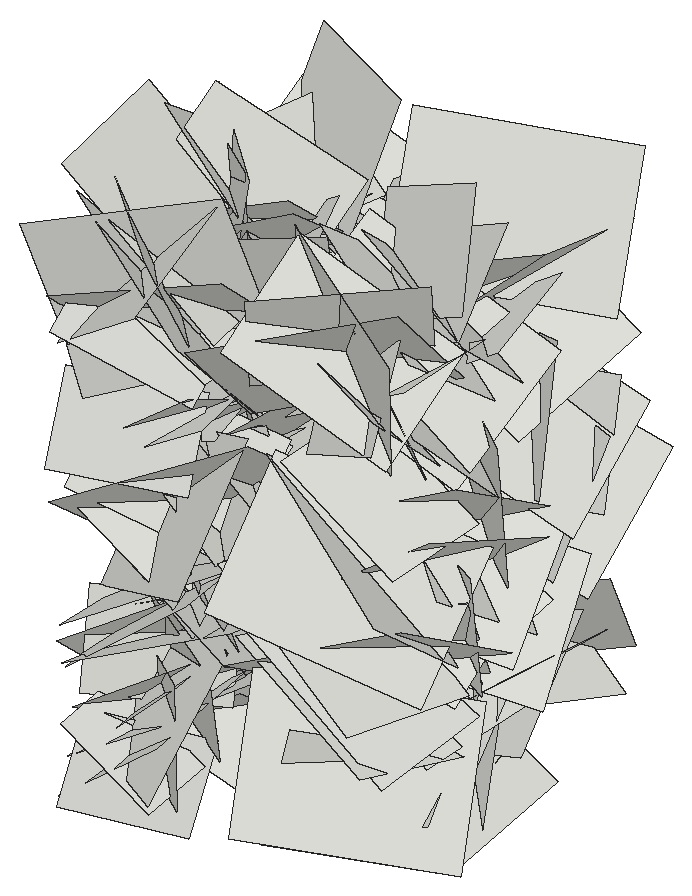
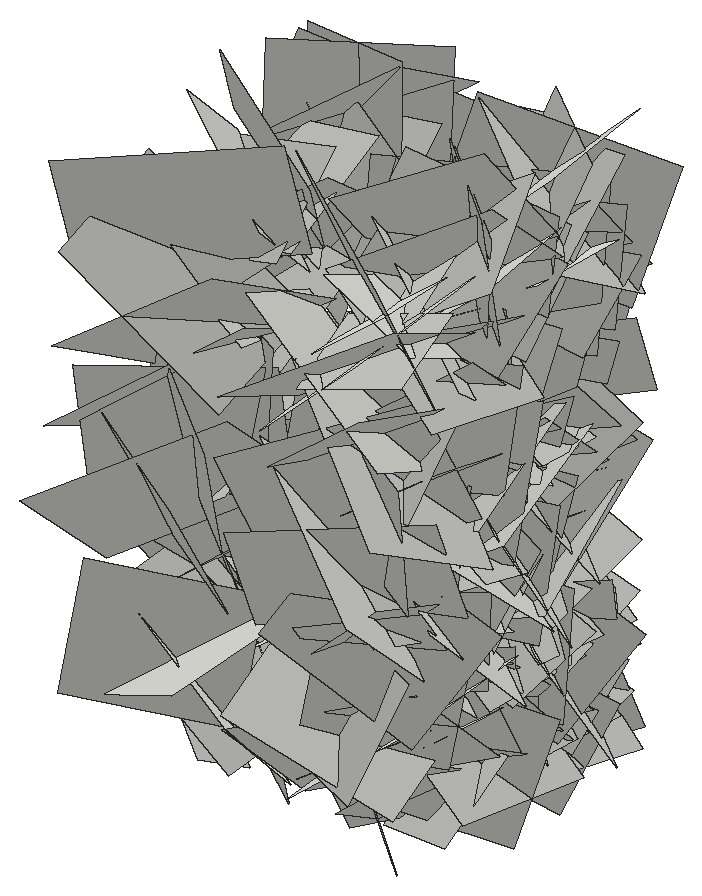
# SketchUp Ruby script. Lengths in inches.
U = 1.inch
M = Sketchup.active_model
def pt(a) = Geom::Point3d.new(a.map { |v| v * U })
def face(e, loops, mat)
  f = e.add_face(loops[0].map { |a| pt(a) })
  loops[1..].each { |l| e.add_face(l.map { |a| pt(a) }).erase! }
  f.material = f.back_material = mat if mat
  f
end
# faces: each face lists its corners as indices into pts; further lists are holes
def faces(e, pts, list, mat = nil) = list.each { |f| face(e, (f[0].is_a?(Array) ? f : [f]).map { |l| l.map { |i| pts[i] } }, mat) }
# xy, xz, yz: faces in a plane at the given z, y or x. An outline is a flat list of corners, or four numbers for a rectangle; further outlines are holes
def ring(l) = l.size == 4 ? [[l[0], l[1]], [l[2], l[1]], [l[2], l[3]], [l[0], l[3]]] : l.each_slice(2).to_a
def flat(e, list, mat, &to3) = list.each { |f| face(e, (f[0].is_a?(Array) ? f : [f]).map { |l| ring(l).map { |u, v| to3.(u, v) } }, mat) }
def xy(e, z, list, mat = nil) = flat(e, list, mat) { |x, y| [x, y, z] }
def xz(e, y, list, mat = nil) = flat(e, list, mat) { |x, z| [x, y, z] }
def yz(e, x, list, mat = nil) = flat(e, list, mat) { |y, z| [x, y, z] }
def lines(e, pts, list) = list.each { |a, b| e.add_line(pt(pts[a]), pt(pts[b])) }
# prism: a flat outline (further loops are holes) pulled along v
def prism(e, loops, v, mat = nil)
  f = face(e, loops, mat); d = Geom::Vector3d.new(v.map { |x| x * U })
  f.pushpull(f.normal.samedirection?(d) ? d.length : -d.length)
end
def box(e, o, s, mat = nil) = prism(e, [[o, [o[0] + s[0], o[1], o[2]], [o[0] + s[0], o[1] + s[1], o[2]], [o[0], o[1] + s[1], o[2]]]], [0, 0, s[2]], mat)
def at(x, y, z, deg = 0) = Geom::Transformation.translation(pt([x, y, z])) * Geom::Transformation.rotation(ORIGIN, Z_AXIS, deg.degrees)
def axes(o, x, y, z) = Geom::Transformation.new([*x, 0, *y, 0, *z, 0, *pt(o).to_a, 1])
def part(name) = M.definitions.add(name)
# library, detail: a bought-in or finely detailed component or shape, given as its bounding box
def library(name, o, s) = part(name).tap { |d| box(d.entities, o, s) }
def detail(e, o, s) = box(e.add_group.entities, o, s)
def put(e, d, t, mat = nil) = e.add_instance(d, t).tap { |i| i.material = mat if mat }
def group(e, t, mat = nil) = e.add_group.tap { |g| g.transformation = t; g.material = mat if mat }.entities
root = M.entities
c1 = part("Component\#6")
p = [[0.01,0,0],[0,3.24,4.54],[4.32,3.24,4.54],[4.33,0,0]]
faces(c1.entities,p,[[0,1,2,3]])
put(root,c1,axes([410.71,188.38,23.95],[-0.14683,-0.05211,-1.06804],[-0.1506,-1.06652,0.07046],[1.12342,-0.14978,-0.13015]))
put(root,c1,axes([414.68,187.95,18.35],[0.24952,-0.85217,0.60628],[0.01294,0.62364,0.87183],[-1.1085,-0.18454,0.14665]))
put(root,c1,axes([414.68,184.68,7.1],[0.07537,-0.21143,-0.85755],[0.01444,-0.85996,0.21315],[-0.93612,-0.03029,-0.06575]))
put(root,c1,axes([410.71,184.16,21.8125],[-0.07155,0.99261,-0.10082],[-0.11355,-0.10768,-0.9884],[1.05147,0.05592,-0.1136]))
put(root,c1,axes([410.71,192.04,5.47],[-0.24252,-0.79203,0.72828],[-0.0092,0.7459,0.80846],[1.14049,-0.1624,0.16139]))
put(root,c1,axes([410.71,189.65,5.54],[0.06955,0.77959,0.08211],[0.00823,0.08175,-0.78235],[0.8309,-0.06607,0.00087]))
put(root,c1,axes([410.71,189.86,21.06],[-0.09411,0.75469,-0.30292],[0.23058,-0.27158,-0.74036],[0.83059,0.16091,0.17121]))
put(root,c1,axes([410.71,184.33,2.33],[-0.23495,-0.78095,0.69461],[0.033,0.70481,0.80235],[1.10738,-0.18669,0.12346]))
put(root,c1,axes([414.68,182.875,15.8],[0.04284,-0.30855,-0.78276],[0.017,-0.78324,0.30957],[-0.8917,-0.02976,-0.0317]))
put(root,c1,axes([414.68,183.91,5.17],[0.1157,0.58195,-0.7538],[0.08085,-0.76164,-0.57696],[-1.0062,0.00571,-0.13304]))
put(root,c1,axes([414.68,180.19,4.07],[-0.08532,0.68038,-0.07405],[-0.04058,-0.07892,-0.68351],[-0.72433,-0.07573,0.04702]))
put(root,c1,axes([414.68,182.98,9.92],[-0.09782,-0.62966,-0.10425],[-0.08997,-0.09229,0.63256],[-0.67052,0.10424,-0.06967]))
put(root,c1,axes([414.68,190.84,12.42],[-0.00848,-0.77925,-0.15089],[0.03038,-0.15108,0.77873],[-0.8408,0.0024,0.02966]))
put(root,c1,axes([414.68,191.35,2.27],[0.06694,-0.86655,-0.10749],[0.04783,-0.10439,0.86806],[-0.92435,-0.06816,0.03713]))
put(root,c1,axes([414.68,191.46,9.82],[0.08538,-0.06629,-0.92063],[0.09555,-0.91915,0.07407],[-0.97372,-0.09601,-0.07345]))
put(root,c1,axes([414.68,193.37,9.31],[0.05697,-0.46717,-0.61186],[-0.09106,-0.61316,0.46062],[-0.81091,0.03603,-0.09471]))
put(root,c1,axes([414.68,183.28,17.73],[0.09647,-0.26045,0.74001],[-0.11879,0.73302,0.27177],[-0.82305,-0.13632,0.04751]))
put(root,c1,axes([414.68,185.14,8.49],[-0.08576,-0.66072,-0.04627],[-0.0456,-0.04128,0.66459],[-0.70059,0.08356,-0.03759]))
put(root,c1,axes([414.68,192.03,8.33],[0.03388,0.22508,-0.86549],[0.13142,-0.8588,-0.21876],[-0.93879,-0.1121,-0.06186]))
put(root,c1,axes([410.71,192.08,20.31],[0.05296,-0.67773,-0.30339],[0.1724,-0.2867,0.66724],[0.76797,0.11109,-0.12886]))
put(root,c1,axes([410.71,184.53,11.29],[-0.10396,-0.95246,0.37472],[-0.04499,0.37989,0.95451],[1.084,-0.07558,0.07555]))
put(root,c1,axes([414.68,183.19,13.8],[0.02762,0.65605,0.3231],[-0.06014,0.32414,-0.6536],[-0.77284,-0.00178,0.06241]))
put(root,c1,axes([414.68,185.94,13.1875],[0.12339,0.16979,-0.82402],[-0.01755,-0.83125,-0.17361],[-0.89164,0.03986,-0.11061]))
put(root,c1,axes([414.68,185.26,12.26],[0.159,0.84642,0.10737],[-0.04855,0.11685,-0.85715],[-0.9031,0.14274,0.06498]))
put(root,c1,axes([410.71,181.6,11.88],[0.05183,0.72565,0.67247],[-0.15864,0.67097,-0.71314],[1.03662,0.0664,-0.14276]))
put(root,c1,axes([414.68,192.38,19.24],[-0.04943,-0.7355,0.057],[0.07325,0.05251,0.73407],[-0.77853,0.05163,0.06545]))
put(root,c1,axes([410.71,185.13,2.21],[0.09174,0.69928,0.36],[0.10121,0.35015,-0.7031],[0.82753,-0.12035,0.04608]))
put(root,c1,axes([410.71,185.25,15.47],[0.04372,0.77316,0.71524],[-0.20224,0.70943,-0.75587],[1.09798,0.09988,-0.16771]))
put(root,c1,axes([410.71,183.61,1.59],[0.06331,-0.78644,0.46242],[-0.03597,0.46118,0.7887],[0.96639,0.06869,-0.00094]))
put(root,c1,axes([410.71,186.63,-0.64],[-0.14781,-0.37723,1.01914],[-0.01271,1.02797,0.37886],[1.15185,-0.03706,0.13496]))
put(root,c1,axes([410.71,183.46,7.83],[-0.1867,0.36795,-0.96583],[0.13041,-0.96532,-0.39019],[1.08777,0.17888,-0.11899]))
put(root,c1,axes([414.68,192.83,7.86],[-0.1126,-0.65912,-0.17655],[0.1088,-0.19208,0.65534],[-0.71507,0.07456,0.12751]))
put(root,c1,axes([414.68,183.375,2.21],[-0.01982,-0.33114,-0.74136],[0.16849,-0.7287,0.32148],[-0.84401,-0.13769,0.08159]))
put(root,c1,axes([410.71,187.85,22.99],[0.09057,-0.06637,-0.91857],[-0.07612,-0.92019,0.05981],[0.97325,-0.06579,0.09016]))
put(root,c1,axes([410.71,187.17,12.95],[-0.05814,-0.16279,1.09674],[-0.14666,1.09051,0.15494],[1.1661,0.12904,0.07417]))
put(root,c1,axes([410.71,185.08,2.16],[0.06404,-1.02262,-0.11109],[-0.17979,-0.11966,1.00929],[1.07543,0.04089,0.17535]))
put(root,c1,axes([410.71,180.14,11.99],[-0.0212,0.75168,0.8023],[-0.17372,0.79143,-0.74558],[1.15236,0.13314,-0.09764]))
put(root,c1,axes([414.68,186.92,8.78],[0.10246,-0.30095,0.75916],[0.04625,0.76527,0.29782],[-0.86439,0.00528,0.10592]))
put(root,c1,axes([410.71,191,16.96],[-0.17643,-1.14926,-0.11809],[-0.05518,-0.11173,1.16072],[1.22339,-0.17078,0.03532]))
put(root,c1,axes([410.71,189.57,16.9],[0.06471,0.53395,-0.71324],[0.01751,-0.71546,-0.53421],[0.94426,-0.02333,0.05878]))
put(root,c1,axes([414.68,184.43,15.42],[0.12844,-0.04329,0.74472],[-0.08874,0.74892,0.05716],[-0.78574,-0.09166,0.11528]))
put(root,c1,axes([410.71,179.97,24.47],[-0.23304,1.36821,0.06434],[-0.25904,0.02493,-1.36533],[1.42861,0.2277,-0.23708]))
put(root,c1,axes([414.68,182.67,1.51],[0.02969,-0.72745,-0.10184],[0.03667,-0.1005,0.72735],[-0.77775,-0.03251,0.03041]))
put(root,c1,axes([410.71,190.33,17.67],[0.17424,0.82504,0.17436],[-0.04616,0.18571,-0.83769],[0.89267,-0.15144,-0.07735]))
put(root,c1,axes([410.71,186.72,4.72],[-0.08241,-0.91883,0.29273],[0.13826,0.28096,0.91654],[1.0128,-0.11312,-0.1013]))
put(root,c1,axes([410.71,185.64,19.96],[-0.2349,1.07139,0.39402],[0.08081,0.41437,-1.08385],[1.20734,0.18072,0.1492]))
put(root,c1,axes([414.68,184.54,3.47],[0.05739,0.5962,-0.42459],[0.0201,-0.42675,-0.59681],[-0.77559,0.03305,-0.04688]))
put(root,c1,axes([414.68,189.45,1.42],[-0.1039,0.30381,0.53974],[0.07033,0.54846,-0.29667],[-0.65275,0.01074,-0.11787]))
put(root,c1,axes([410.71,186.9375,3.03],[0.11563,0.62873,-0.58509],[0.05581,-0.59358,-0.62803],[0.90867,-0.04354,0.11303]))
put(root,c1,axes([410.71,184.51,1.15],[-0.01173,-1.06899,-0.22188],[-0.10644,-0.21996,1.06472],[1.15237,-0.0312,0.09608]))
put(root,c1,axes([414.68,183.83,7.3125],[0.02805,0.62389,-0.09529],[-0.05665,-0.09282,-0.62253],[-0.66659,0.03414,0.0489]))
put(root,c1,axes([414.68,183.1,18.89],[0.1435,0.17311,-0.85276],[0.14536,-0.85648,-0.1521],[-0.91084,-0.10941,-0.15862]))
put(root,c1,axes([410.71,187.61,11.62],[-0.28203,-0.58282,-1.12773],[0.01249,-1.15332,0.59327],[1.34554,-0.11146,-0.24188]))
put(root,c1,axes([410.71,184.19,13.53],[0.08078,-0.49886,0.79857],[0.01528,0.8017,0.49945],[0.99796,0.02811,-0.07229]))
put(root,c1,axes([410.71,181.29,16.68],[0.08133,-0.245,0.96212],[-0.05676,0.96256,0.24939],[1.05086,0.07095,-0.06099]))
put(root,c1,axes([414.68,186.0625,6.1],[0.08854,0.52684,0.45627],[-0.00383,0.45985,-0.53032],[-0.73876,0.06076,0.05744]))
put(root,c1,axes([414.68,187.98,11.49],[0.12716,0.81746,0.20835],[0.15,0.18797,-0.81896],[-0.88154,0.1499,-0.10929]))
put(root,c1,axes([410.71,194.3,13.93],[-0.22437,-1.23478,-0.60854],[-0.19245,-0.58527,1.25072],[1.44644,-0.26941,0.07201]))
put(root,c1,axes([410.71,184.41,20.14],[-0.03821,-1.03167,-0.60174],[-0.15497,-0.59368,1.0266],[1.25647,-0.1046,0.10832]))
put(root,c1,axes([414.68,186.3,8.38],[-0.07617,0.47932,0.41871],[0.13681,0.42359,-0.46276],[-0.66062,0.03245,-0.14411]))
put(root,c1,axes([410.71,184.31,4.6],[0.1576,-0.1516,-1.0147],[-0.15202,-1.0183,0.13112],[1.07684,-0.12157,0.16702]))
put(root,c1,axes([410.71,179.32,18.3],[0.15069,0.54422,0.74866],[-0.00735,0.75804,-0.54972],[0.98107,-0.07791,-0.11911]))
put(root,c1,axes([414.68,188.8,6.44],[0.14743,-0.18272,-0.74199],[0.06403,-0.74919,0.19581],[-0.80747,-0.09277,-0.11994]))
put(root,c1,axes([410.71,185.52,6.2],[-0.2751,-0.65276,-1.16933],[-0.03559,-1.18754,0.67037],[1.41909,-0.15632,-0.20987]))
put(root,c1,axes([410.71,181.08,20.02],[-0.00536,1.00575,0.03656],[0.10796,0.03689,-1.00058],[1.06133,0.00133,0.10197]))
put(root,c1,axes([410.71,184.05,20.67],[0.10102,0.73684,0.6989],[-0.04073,0.70408,-0.73707],[1.07574,-0.04254,-0.09354]))
put(root,c1,axes([410.71,191.125,9.45],[-0.23474,-0.88576,-0.93612],[0.00151,-0.95001,0.89856],[1.36608,-0.15116,-0.16185]))
put(root,c1,axes([410.71,185.11,13.22],[0.08906,-0.95701,-0.12674],[0.0585,-0.12225,0.95969],[1.02162,0.09043,-0.0439]))
put(root,c1,axes([410.71,180.4,17.125],[-0.23878,-0.31981,1.17522],[0.15258,1.17979,0.34864],[1.28199,-0.19998,0.17739]))
put(root,c1,axes([410.71,187.48,17.59],[-0.04794,-0.78864,0.66349],[0.19289,0.64758,0.78214],[1.07529,-0.15133,-0.11072]))
put(root,c1,axes([410.71,187.26,9.21],[0.06299,-0.71122,-0.64775],[0.16214,-0.63375,0.70987],[1.00673,0.14657,-0.0738]))
put(root,c1,axes([414.68,191.11,1.26],[0.04561,-0.57908,-0.31344],[0.1156,-0.3035,0.57569],[-0.68833,-0.08935,0.07592]))
put(root,c1,axes([410.71,186.13,19.34],[0.13168,0.96657,0.23982],[0.01085,0.24043,-0.97432],[1.05558,-0.12304,-0.0199]))
put(root,c1,axes([410.71,188.68,19.83],[-0.08458,1.11358,0.50301],[-0.01593,0.50315,-1.11627],[1.29513,0.07891,0.01912]))
put(root,c1,axes([410.71,185.36,5.79],[0.02078,-1.22604,-0.15411],[-0.11589,-0.15525,1.22117],[1.3047,0.00574,0.11093]))
put(root,c1,axes([410.71,186.43,6.6],[-0.00451,1.27416,-0.10814],[-0.14001,-0.108,-1.26731],[1.34821,-0.00695,-0.13197]))
put(root,c1,axes([414.68,190.35,18.26],[0.16101,-0.65287,0.16772],[0.08445,0.18811,0.66008],[-0.7095,-0.12576,0.11663]))
put(root,c1,axes([410.71,187.9375,5.11],[0.04973,-1.23753,-0.07043],[-0.13139,-0.07481,1.23194],[1.30732,0.03956,0.12649]))
put(root,c1,axes([410.71,189.08,9.2],[-0.13088,0.55221,1.09741],[0.12619,1.10312,-0.54169],[1.29609,-0.05164,0.16356]))
put(root,c1,axes([410.71,182.44,13.63],[-0.1579,1.28482,-0.45217],[-0.02165,-0.45692,-1.2916],[1.44363,0.13368,-0.06883]))
put(root,c1,axes([410.71,182.53,23.48],[0.24403,0.37129,-0.99391],[-0.1038,-1.00526,-0.39821],[1.11985,-0.17408,0.17968]))
put(root,c1,axes([410.71,192.17,8.01],[0.17438,0.53527,-0.89237],[0.02164,-0.90494,-0.53904],[1.10282,-0.06688,0.15168]))
put(root,c1,axes([410.71,188.23,7.57],[0.0913,-1.12353,0.75234],[-0.27462,0.72618,1.11413],[1.40673,0.21468,0.16867]))
put(root,c1,axes([410.71,194.04,23.84],[-0.15699,-0.54259,-1.24113],[0.03696,-1.24964,0.54215],[1.43535,-0.02717,-0.14971]))
put(root,c1,axes([410.71,189.36,1.43],[-0.09807,-1.35815,-0.14277],[-0.05055,-0.1398,1.36078],[1.44669,-0.09695,0.03787]))
put(root,c1,axes([410.71,188.7,21.97],[0.14471,1.28216,-0.28655],[-0.25359,-0.25902,-1.27293],[1.36933,-0.18346,-0.20546]))
put(root,c1,axes([410.71,190.12,11.53],[-0.21117,-0.99907,-0.90649],[0.1512,-0.92678,0.99009],[1.42194,-0.04983,-0.2399]))
put(root,c1,axes([410.71,183.02,16.38],[-0.02893,-0.8566,0.75588],[0.26219,0.73373,0.84043],[1.18223,-0.18368,-0.16789]))
put(root,c1,axes([410.71,185.31,6.45],[-0.03902,-0.20515,1.15818],[0.22164,1.13915,0.20842],[1.22693,-0.21231,-0.00082]))
put(root,c1,axes([410.71,180.93,10.86],[-0.17521,1.15715,-0.62152],[0.20897,-0.59747,-1.1648],[1.37654,0.23798,0.09772]))
put(root,c1,axes([410.71,184.5,10.44],[0.20009,0.552,-0.98447],[-0.02572,-0.99592,-0.56307],[1.1961,-0.11375,0.15258]))
put(root,c1,axes([410.71,185.25,0.97],[0.15144,0.45294,1.0525],[0.02813,1.05906,-0.45936],[1.21425,-0.08102,-0.12063]))
put(root,c1,axes([410.71,182.38,2.76],[0.16715,0.82367,0.72398],[0.09449,0.71938,-0.83785],[1.15857,-0.1775,-0.03612]))
put(root,c1,axes([410.71,186.66,10.07],[-0.09303,-0.2424,1.37134],[-0.00293,1.37409,0.24271],[1.47615,-0.01254,0.08691]))
put(root,c1,axes([410.71,192.77,15.58],[0.03721,-0.16955,-1.17702],[0.1418,-1.1695,0.17246],[1.25252,0.13744,0.01545]))
put(root,c1,axes([410.71,185.87,11.99],[0.00632,-0.88407,-1.06115],[-0.10628,-1.05864,0.88141],[1.46017,-0.07323,0.06874]))
put(root,c1,axes([410.71,186.02,17.55],[0.12484,-0.91824,0.67786],[0.09261,0.68671,0.91505],[1.20627,0.04231,-0.14041]))
put(root,c1,axes([410.71,195.54,11.625],[0.04246,-1.00606,-0.92627],[-0.11693,-0.92602,1.00103],[1.44486,-0.04538,0.10823]))
put(root,c1,axes([410.71,183.88,15.08],[-0.0404,1.11797,-0.62329],[0.16276,-0.61507,-1.11262],[1.34698,0.10785,0.11575]))
put(root,c1,axes([410.71,184.23,21.55],[0.30098,0.54789,0.85036],[0.10123,0.86476,-0.58905],[1.06749,-0.23649,-0.1839]))
put(root,c1,axes([410.71,184,8.18],[-0.02134,-1.06466,0.81449],[0.04088,0.81378,1.06469],[1.42032,-0.03942,-0.01841]))
put(root,c1,axes([410.71,188.34,12.62],[0.20954,0.481,1.15591],[-0.07101,1.17261,-0.47649],[1.32521,-0.01322,-0.2083]))
put(root,c1,axes([410.71,186.39,13.5625],[0.22643,-0.80881,0.81079],[0.0736,0.83241,0.81208],[1.21171,0.10058,-0.20084]))
put(root,c1,axes([410.71,184.34,4.6],[0.11485,-1.15497,0.26483],[0.19184,0.27894,1.14248],[1.2413,0.06375,-0.20107]))
put(root,c1,axes([410.71,193.03,3.2],[0.23388,-1.096,0.27231],[0.13541,0.2999,1.10354],[1.1894,0.18138,-0.17918]))
put(root,c1,axes([410.71,189.55,17.94],[0.16397,-1.09761,-0.83604],[-0.11999,-0.84854,1.09307],[1.45761,0.05363,0.18403]))
put(root,c1,axes([410.71,187.39,3.1875],[0.10139,0.89849,0.89189],[0.1671,0.87902,-0.90243],[1.33152,-0.17873,0.04534]))
put(root,c1,axes([410.71,180.76,23.09],[0.06995,0.91309,-0.96842],[0.10566,-0.97028,-0.90805],[1.4069,0.02747,0.11634]))
put(root,c1,axes([410.71,183.54,2.14],[0.03864,0.84179,0.92004],[0.33491,0.88417,-0.82148],[1.27872,-0.257,0.18735]))
put(root,c1,axes([410.71,184.58,6.82],[0.16596,-1.29847,0.14138],[0.0614,0.14916,1.30572],[1.38315,0.14917,-0.07492]))
put(root,c1,axes([410.71,193.85,16.74],[0.30124,-1.14539,-0.57535],[-0.00001,-0.58933,1.17321],[1.35869,0.25394,0.12757]))
put(root,c1,axes([410.71,189.11,8.53],[0.25892,-1.11224,-0.53402],[0.14932,-0.51568,1.13849],[1.29927,0.28091,-0.02442]))
put(root,c1,axes([410.71,182.27,16.13],[0.23771,-0.47409,1.27281],[0.00404,1.29026,0.47991],[1.43973,0.07465,-0.2115]))
put(root,c1,axes([424.49,182.27,16.13],[-0.23771,-0.47409,1.27281],[-0.00404,1.29026,0.47991],[-1.43973,0.07465,-0.2115]))
put(root,c1,axes([424.49,189.11,8.53],[-0.25892,-1.11224,-0.53402],[-0.14932,-0.51568,1.13849],[-1.29927,0.28091,-0.02442]))
put(root,c1,axes([424.49,193.85,16.74],[-0.30124,-1.14539,-0.57535],[0.00001,-0.58933,1.17321],[-1.35869,0.25394,0.12757]))
put(root,c1,axes([424.49,184.58,6.82],[-0.16596,-1.29847,0.14138],[-0.0614,0.14916,1.30572],[-1.38315,0.14917,-0.07492]))
put(root,c1,axes([424.49,183.54,2.14],[-0.03864,0.84179,0.92004],[-0.33491,0.88417,-0.82148],[-1.27872,-0.257,0.18735]))
put(root,c1,axes([424.49,180.76,23.09],[-0.06995,0.91309,-0.96842],[-0.10566,-0.97028,-0.90805],[-1.4069,0.02747,0.11634]))
put(root,c1,axes([424.49,187.39,3.1875],[-0.10139,0.89849,0.89189],[-0.1671,0.87902,-0.90243],[-1.33152,-0.17873,0.04534]))
put(root,c1,axes([424.49,189.55,17.94],[-0.16397,-1.09761,-0.83604],[0.11999,-0.84854,1.09307],[-1.45761,0.05363,0.18403]))
put(root,c1,axes([424.49,193.03,3.2],[-0.23388,-1.096,0.27231],[-0.13541,0.2999,1.10354],[-1.1894,0.18138,-0.17918]))
put(root,c1,axes([424.49,184.34,4.6],[-0.11485,-1.15497,0.26483],[-0.19184,0.27894,1.14248],[-1.2413,0.06375,-0.20107]))
put(root,c1,axes([424.49,186.39,13.5625],[-0.22643,-0.80881,0.81079],[-0.0736,0.83241,0.81208],[-1.21171,0.10058,-0.20084]))
put(root,c1,axes([424.49,188.34,12.62],[-0.20954,0.481,1.15591],[0.07101,1.17261,-0.47649],[-1.32521,-0.01322,-0.2083]))
put(root,c1,axes([424.49,184,8.18],[0.02134,-1.06466,0.81449],[-0.04088,0.81378,1.06469],[-1.42032,-0.03942,-0.01841]))
put(root,c1,axes([424.49,184.23,21.55],[-0.30098,0.54789,0.85036],[-0.10123,0.86476,-0.58905],[-1.06749,-0.23649,-0.1839]))
put(root,c1,axes([424.49,183.88,15.08],[0.0404,1.11797,-0.62329],[-0.16276,-0.61507,-1.11262],[-1.34698,0.10785,0.11575]))
put(root,c1,axes([424.49,195.54,11.625],[-0.04246,-1.00606,-0.92627],[0.11693,-0.92602,1.00103],[-1.44486,-0.04538,0.10823]))
put(root,c1,axes([424.49,186.02,17.55],[-0.12484,-0.91824,0.67786],[-0.09261,0.68671,0.91505],[-1.20627,0.04231,-0.14041]))
put(root,c1,axes([424.49,185.87,11.99],[-0.00632,-0.88407,-1.06115],[0.10628,-1.05864,0.88141],[-1.46017,-0.07323,0.06874]))
put(root,c1,axes([424.49,192.77,15.58],[-0.03721,-0.16955,-1.17702],[-0.1418,-1.1695,0.17246],[-1.25252,0.13744,0.01545]))
put(root,c1,axes([424.49,186.66,10.07],[0.09303,-0.2424,1.37134],[0.00293,1.37409,0.24271],[-1.47615,-0.01254,0.08691]))
put(root,c1,axes([424.49,182.38,2.76],[-0.16715,0.82367,0.72398],[-0.09449,0.71938,-0.83785],[-1.15857,-0.1775,-0.03612]))
put(root,c1,axes([424.49,185.25,0.97],[-0.15144,0.45294,1.0525],[-0.02813,1.05906,-0.45936],[-1.21425,-0.08102,-0.12063]))
put(root,c1,axes([424.49,184.5,10.44],[-0.20009,0.552,-0.98447],[0.02572,-0.99592,-0.56307],[-1.1961,-0.11375,0.15258]))
put(root,c1,axes([424.49,180.93,10.86],[0.17521,1.15715,-0.62152],[-0.20897,-0.59747,-1.1648],[-1.37654,0.23798,0.09772]))
put(root,c1,axes([424.49,185.31,6.45],[0.03902,-0.20515,1.15818],[-0.22164,1.13915,0.20842],[-1.22693,-0.21231,-0.00082]))
put(root,c1,axes([424.49,183.02,16.38],[0.02893,-0.8566,0.75588],[-0.26219,0.73373,0.84043],[-1.18223,-0.18368,-0.16789]))
put(root,c1,axes([424.49,190.12,11.53],[0.21117,-0.99907,-0.90649],[-0.1512,-0.92678,0.99009],[-1.42194,-0.04983,-0.2399]))
put(root,c1,axes([424.49,188.7,21.97],[-0.14471,1.28216,-0.28655],[0.25359,-0.25902,-1.27293],[-1.36933,-0.18346,-0.20546]))
put(root,c1,axes([424.49,189.36,1.43],[0.09807,-1.35815,-0.14277],[0.05055,-0.1398,1.36078],[-1.44669,-0.09695,0.03787]))
put(root,c1,axes([424.49,194.04,23.84],[0.15699,-0.54259,-1.24113],[-0.03696,-1.24964,0.54215],[-1.43535,-0.02717,-0.14971]))
put(root,c1,axes([424.49,188.23,7.57],[-0.0913,-1.12353,0.75234],[0.27462,0.72618,1.11413],[-1.40673,0.21468,0.16867]))
put(root,c1,axes([424.49,192.17,8.01],[-0.17438,0.53527,-0.89237],[-0.02164,-0.90494,-0.53904],[-1.10282,-0.06688,0.15168]))
put(root,c1,axes([424.49,182.53,23.48],[-0.24403,0.37129,-0.99391],[0.1038,-1.00526,-0.39821],[-1.11985,-0.17408,0.17968]))
put(root,c1,axes([424.49,182.44,13.63],[0.1579,1.28482,-0.45217],[0.02165,-0.45692,-1.2916],[-1.44363,0.13368,-0.06883]))
put(root,c1,axes([424.49,189.08,9.2],[0.13088,0.55221,1.09741],[-0.12619,1.10312,-0.54169],[-1.29609,-0.05164,0.16356]))
put(root,c1,axes([424.49,187.9375,5.11],[-0.04973,-1.23753,-0.07043],[0.13139,-0.07481,1.23194],[-1.30732,0.03956,0.12649]))
put(root,c1,axes([420.52,190.35,18.26],[-0.16101,-0.65287,0.16772],[-0.08445,0.18811,0.66008],[0.7095,-0.12576,0.11663]))
put(root,c1,axes([424.49,186.43,6.6],[0.00451,1.27416,-0.10814],[0.14001,-0.108,-1.26731],[-1.34821,-0.00695,-0.13197]))
put(root,c1,axes([424.49,185.36,5.79],[-0.02078,-1.22604,-0.15411],[0.11589,-0.15525,1.22117],[-1.3047,0.00574,0.11093]))
put(root,c1,axes([424.49,186.13,19.34],[-0.13168,0.96657,0.23982],[-0.01085,0.24043,-0.97432],[-1.05558,-0.12304,-0.0199]))
put(root,c1,axes([420.52,191.11,1.26],[-0.04561,-0.57908,-0.31344],[-0.1156,-0.3035,0.57569],[0.68833,-0.08935,0.07592]))
put(root,c1,axes([424.49,187.26,9.21],[-0.06299,-0.71122,-0.64775],[-0.16214,-0.63375,0.70987],[-1.00673,0.14657,-0.0738]))
put(root,c1,axes([424.49,187.48,17.59],[0.04794,-0.78864,0.66349],[-0.19289,0.64758,0.78214],[-1.07529,-0.15133,-0.11072]))
put(root,c1,axes([424.49,180.4,17.125],[0.23878,-0.31981,1.17522],[-0.15258,1.17979,0.34864],[-1.28199,-0.19998,0.17739]))
put(root,c1,axes([424.49,185.11,13.22],[-0.08906,-0.95701,-0.12674],[-0.0585,-0.12225,0.95969],[-1.02162,0.09043,-0.0439]))
put(root,c1,axes([424.49,191.125,9.45],[0.23474,-0.88576,-0.93612],[-0.00151,-0.95001,0.89856],[-1.36608,-0.15116,-0.16185]))
put(root,c1,axes([424.49,184.05,20.67],[-0.10102,0.73684,0.6989],[0.04073,0.70408,-0.73707],[-1.07574,-0.04254,-0.09354]))
put(root,c1,axes([424.49,181.08,20.02],[0.00536,1.00575,0.03656],[-0.10796,0.03689,-1.00058],[-1.06133,0.00133,0.10197]))
put(root,c1,axes([424.49,185.52,6.2],[0.2751,-0.65276,-1.16933],[0.03559,-1.18754,0.67037],[-1.41909,-0.15632,-0.20987]))
put(root,c1,axes([420.52,188.8,6.44],[-0.14743,-0.18272,-0.74199],[-0.06403,-0.74919,0.19581],[0.80747,-0.09277,-0.11994]))
put(root,c1,axes([424.49,179.32,18.3],[-0.15069,0.54422,0.74866],[0.00735,0.75804,-0.54972],[-0.98107,-0.07791,-0.11911]))
put(root,c1,axes([424.49,184.31,4.6],[-0.1576,-0.1516,-1.0147],[0.15202,-1.0183,0.13112],[-1.07684,-0.12157,0.16702]))
put(root,c1,axes([420.52,186.3,8.38],[0.07617,0.47932,0.41871],[-0.13681,0.42359,-0.46276],[0.66062,0.03245,-0.14411]))
put(root,c1,axes([424.49,184.41,20.14],[0.03821,-1.03167,-0.60174],[0.15497,-0.59368,1.0266],[-1.25647,-0.1046,0.10832]))
put(root,c1,axes([424.49,194.3,13.93],[0.22437,-1.23478,-0.60854],[0.19245,-0.58527,1.25072],[-1.44644,-0.26941,0.07201]))
